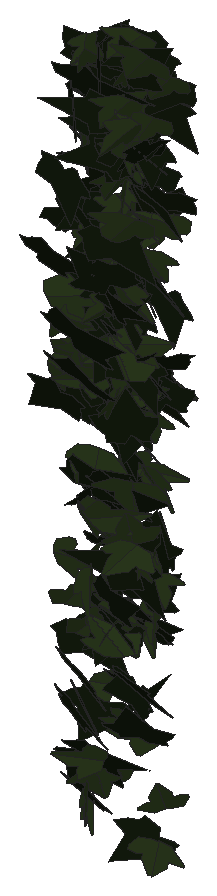
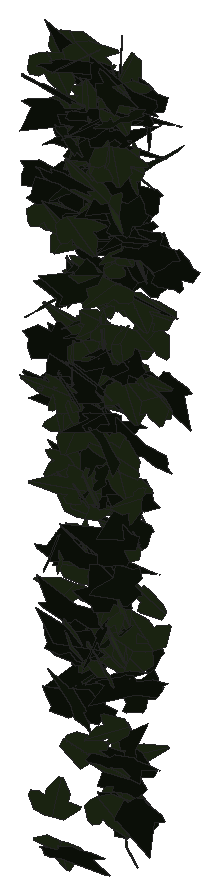
# SketchUp Ruby script. Lengths in millimetres.
U = 1.mm
M = Sketchup.active_model
def pt(a) = Geom::Point3d.new(a.map { |v| v * U })
def face(e, loops, mat)
  f = e.add_face(loops[0].map { |a| pt(a) })
  loops[1..].each { |l| e.add_face(l.map { |a| pt(a) }).erase! }
  f.material = f.back_material = mat if mat
  f
end
# faces: each face lists its corners as indices into pts; further lists are holes
def faces(e, pts, list, mat = nil) = list.each { |f| face(e, (f[0].is_a?(Array) ? f : [f]).map { |l| l.map { |i| pts[i] } }, mat) }
# xy, xz, yz: faces in a plane at the given z, y or x. An outline is a flat list of corners, or four numbers for a rectangle; further outlines are holes
def ring(l) = l.size == 4 ? [[l[0], l[1]], [l[2], l[1]], [l[2], l[3]], [l[0], l[3]]] : l.each_slice(2).to_a
def flat(e, list, mat, &to3) = list.each { |f| face(e, (f[0].is_a?(Array) ? f : [f]).map { |l| ring(l).map { |u, v| to3.(u, v) } }, mat) }
def xy(e, z, list, mat = nil) = flat(e, list, mat) { |x, y| [x, y, z] }
def xz(e, y, list, mat = nil) = flat(e, list, mat) { |x, z| [x, y, z] }
def yz(e, x, list, mat = nil) = flat(e, list, mat) { |y, z| [x, y, z] }
def lines(e, pts, list) = list.each { |a, b| e.add_line(pt(pts[a]), pt(pts[b])) }
# prism: a flat outline (further loops are holes) pulled along v
def prism(e, loops, v, mat = nil)
  f = face(e, loops, mat); d = Geom::Vector3d.new(v.map { |x| x * U })
  f.pushpull(f.normal.samedirection?(d) ? d.length : -d.length)
end
def box(e, o, s, mat = nil) = prism(e, [[o, [o[0] + s[0], o[1], o[2]], [o[0] + s[0], o[1] + s[1], o[2]], [o[0], o[1] + s[1], o[2]]]], [0, 0, s[2]], mat)
def at(x, y, z, deg = 0) = Geom::Transformation.translation(pt([x, y, z])) * Geom::Transformation.rotation(ORIGIN, Z_AXIS, deg.degrees)
def axes(o, x, y, z) = Geom::Transformation.new([*x, 0, *y, 0, *z, 0, *pt(o).to_a, 1])
def part(name) = M.definitions.add(name)
# library, detail: a bought-in or finely detailed component or shape, given as its bounding box
def library(name, o, s) = part(name).tap { |d| box(d.entities, o, s) }
def detail(e, o, s) = box(e.add_group.entities, o, s)
def put(e, d, t, mat = nil) = e.add_instance(d, t).tap { |i| i.material = mat if mat }
def group(e, t, mat = nil) = e.add_group.tap { |g| g.transformation = t; g.material = mat if mat }.entities
root = M.entities
M.materials.add("efeu1").color = [18, 25, 13]
M.materials.add("efeu2").color = [43, 57, 29]
c1 = part("ivyleaf_9")
p = [[39.1,54.8,31.7],[34.5,51.8,30.2],[-5.3,25.2,17.3],[-17.9,28.3,20.9],[-21.6,21.7,17],[-20.2,4.3,5.3],
  [-22.9,-0.3,2.5],[-17.1,-4,-0.6],[-2,-2.1,-1.2],[-0.7,-15.4,-10.1],[16.6,-22.3,-16.7],[21.1,-15.1,-12.5],
  [32.7,-10.7,-11],[46.1,-1.8,-6.6],[30.8,11.2,3.8]]
faces(c1.entities,p,[[0,1,2,3,4,5,6,7,8,9,10,11,12,13,14]],"efeu1")
c2 = part("ivyleaf_10")
p = [[0,12.8,-0.8],[-1.5,51.3,-10.9],[-4.9,51,-11.6],[-13.6,26.5,-7.3],[-13.2,15.9,-4.6],[-21.1,19.3,-7.2],
  [-29.5,16.3,-8.3],[-29.2,8.3,-6.2],[-19.7,-9.8,0.5],[-7.6,-13,4],[1,-12.2,5.8],[-0.4,51.1,-11.1],
  [-1.5,51.1,-10.9],[1,-12.4,5.9],[16.9,-12.4,3.5],[35.1,9.1,-5.1],[35,12.9,-6.1],[20.5,16.4,-4.9],
  [15.8,15,-3.8],[15.3,27.6,-7.1],[12.8,31.3,-7.8]]
faces(c2.entities,p,[[0,1,2,3,4,5,6,7,8,9,10],[11,12,0,13,14,15,16,17,18,19,20]],"efeu2")
put(root,c1,axes([2636.7,760.3,1184.7],[1.6124,-0.56615,0.10588],[-0.16714,0.05915,1.01896],[-1.08336,-0.85174,0.00038]))
put(root,c1,axes([2611.5,780.2,1231.1],[-0.08714,-0.29377,1.10403],[1.30837,-0.88957,-0.20819],[1.73659,0.65547,0.21226]))
put(root,c2,axes([2633.5,781.2,864.3],[0.85683,-0.49021,0.75163],[0.95653,-0.55892,-0.66555],[1.41486,0.67472,-0.00523]))
put(root,c1,axes([2588.5,792.1,648.9],[1.43319,-0.52934,-0.36142],[-0.54841,0.2185,-0.92039],[1.08964,0.8062,0.01214]))
put(root,c2,axes([2649.6,821.7,1130.2],[0.1327,-0.81984,-0.18916],[-0.03294,0.18837,-0.8228],[1.60097,0.07183,-0.00125]))
put(root,c1,axes([2544.3,843.4,1440.8],[-0.05269,-0.95204,0.27297],[-0.03417,-0.27255,-0.95239],[1.88462,-0.03156,-0.00964]))
put(root,c1,axes([2544.1,833.4,1099.3],[0.62412,0.12421,-0.75032],[-1.35263,-0.24082,-0.35049],[-0.51525,0.78264,0.01124]))
put(root,c2,axes([2661,844.7,884.5],[1.00057,0.45595,-0.51321],[-0.72793,-0.34225,-0.69588],[-1.08498,0.65011,-0.00641]))
put(root,c2,axes([2648.4,855.7,1540],[-0.23392,-0.64575,0.69785],[-0.07905,-0.69934,-0.65444],[1.80781,-0.11414,0.06168]))
put(root,c2,axes([2657.9,846.9,1398.1],[-1.29079,-0.56031,0.38123],[-0.57404,-0.23343,-0.87966],[1.15502,-0.74218,-0.01114]))
put(root,c1,axes([2613.9,854.3,1285.2],[0.65721,0.16862,0.86839],[-1.60064,-0.22643,0.3784],[0.52195,-0.90669,0.06699]))
put(root,c1,axes([2665.8,837.4,1077.4],[-1.67349,0.36104,-0.12202],[-0.22886,0.02832,0.95034],[0.68826,0.88728,0.01932]))
put(root,c1,axes([2620.6,846.9,1370.6],[0.06708,-0.68505,-0.71505],[0.24385,0.71265,-0.67643],[1.8688,-0.0684,0.11393]))
put(root,c1,axes([2492.5,858.1,1287.3],[0.42343,-0.24255,0.75106],[1.05325,-0.50842,-0.32813],[1.07097,0.5959,0.02575]))
put(root,c2,axes([2622.8,869.5,1114.2],[0.05493,-0.1984,0.87429],[0.54078,-0.82763,-0.19719],[1.6183,0.2833,0.03622]))
put(root,c2,axes([2580,865.8,518.5],[-0.23204,-0.13674,-0.84716],[-1.16666,-0.5849,0.18263],[-1.14288,0.62484,-0.01444]))
put(root,c2,axes([2563,867,463.3],[0.47772,-0.50253,0.66321],[0.81387,-0.51635,-0.55309],[1.35852,0.48605,0.09813]))
put(root,c1,axes([2587.5,870.7,1246.5],[0.35757,-0.24664,0.81519],[0.86605,-0.67658,-0.30958],[1.37018,0.49202,-0.01706]))
put(root,c2,axes([2573.1,872.8,1113.6],[0.33756,0.20389,-0.77068],[-1.33007,-0.3401,-0.25081],[-0.72999,0.71396,0.10061]))
put(root,c2,axes([2640.6,875.7,884.5],[-0.95042,-0.75998,-0.32042],[-0.33718,-0.26699,0.90937],[-1.53305,0.52987,-0.00136]))
put(root,c2,axes([2600,857.9,908.2],[-0.4951,-0.32007,0.79563],[0.97281,0.60975,0.41242],[-1.3106,0.57351,0.00556]))
put(root,c2,axes([2636.8,865.7,1150.4],[1.45285,0.14221,0.28272],[-0.54953,0.01077,0.77421],[0.24656,-0.81397,0.05964]))
put(root,c1,axes([2595.3,880.6,765.3],[-0.07981,-0.01194,0.86813],[0.66293,-0.79636,0.00587],[1.51356,0.34817,0.0432]))
put(root,c2,axes([2594.9,884.7,1234],[-0.18894,-0.47209,0.65973],[-0.19717,-0.65183,-0.48203],[1.53131,-0.14218,0.01934]))
put(root,c1,axes([2611.1,884.4,1469.2],[-1.27105,-0.07874,0.49317],[-0.88576,-0.20058,-0.66228],[0.34477,-0.80561,0.11669]))
put(root,c1,axes([2665.5,864.2,1102.1],[-0.0001,0.82108,0.13207],[0.00018,0.13207,-0.82108],[-1.58276,-0.00004,-0.0001]))
put(root,c2,axes([2498.8,885.8,1100.2],[-0.08474,-0.04414,-0.80849],[1.05544,-0.59165,0.00176],[-1.12284,-0.5528,0.06267]))
put(root,c1,axes([2524.4,889.7,635.8],[0.49437,-0.66612,0.54837],[0.3917,-0.50832,-0.71495],[1.59468,0.33136,0.00561]))
put(root,c2,axes([2609.1,878,701.1],[1.07533,0.55125,0.36674],[-0.5215,-0.24422,0.78923],[1.14713,-0.62777,0.01501]))
put(root,c1,axes([2518.9,889.7,1539],[-0.20167,0.03786,-0.92487],[1.53236,-0.4555,-0.11089],[-0.86914,-0.81187,0.01908]))
put(root,c1,axes([2600.6,892.9,1242.9],[-0.12424,-0.10747,0.81775],[-0.65781,-0.74124,-0.12501],[1.42525,-0.35148,0.01359]))
put(root,c1,axes([2641.9,883.7,572],[1.28895,-0.00393,0.47864],[-0.9109,0.0059,0.67726],[-0.01259,-0.8293,0.00255]))
put(root,c1,axes([2627.8,895.5,631.9],[0.61513,-0.71398,-0.4213],[0.31013,-0.38865,0.78366],[-1.54699,-0.36181,-0.01042]))
put(root,c1,axes([2636.2,883.3,1158.1],[-0.16363,-0.83193,-0.3462],[0.0873,0.34328,-0.83631],[1.71274,-0.09698,0.00956]))
put(root,c1,axes([2614.1,898.9,1050.6],[-0.30402,-0.84049,0.4832],[-0.08675,-0.48266,-0.85462],[1.84308,-0.16136,0.03948]))
put(root,c2,axes([2614.8,888.1,1551.9],[-0.81112,-0.66346,0.40932],[-0.30664,-0.38146,-0.78606],[1.45163,-0.45129,0.06267]))
put(root,c2,axes([2637.9,879.6,962.2],[-1.64954,-0.50452,-0.01723],[0.03126,0.00604,-1.00286],[0.96025,-0.86687,0.00304]))
put(root,c2,axes([2615.9,886.7,1261.3],[-0.83842,0.17875,-0.66675],[1.00765,-0.42003,-0.46243],[-0.84299,-0.67985,0.11039]))
put(root,c2,axes([2515,872.2,1224.9],[0.4771,0.06473,-0.91337],[1.62568,0.3246,0.25744],[0.62777,-0.88978,0.02747]))
put(root,c1,axes([2591.7,887.1,1526],[-0.97841,0.14637,0.63984],[-1.24803,-0.07931,-0.50873],[-0.05415,-0.81694,0.16403]))
put(root,c2,axes([2538.2,894.7,1469.3],[-0.2072,0.51045,-0.77588],[0.32854,-0.75646,-0.52189],[-1.73677,-0.20399,-0.00616]))
put(root,c1,axes([2552.9,894.8,877.4],[0.44546,-0.56495,0.55341],[0.4044,-0.51099,-0.61151],[1.44979,0.31612,0.00053]))
put(root,c1,axes([2594.9,890,928.6],[-0.04633,-0.21976,0.96131],[1.4186,-0.63368,-0.12599],[1.22875,0.7233,0.1817]))
put(root,c1,axes([2626.7,889.4,824.4],[-0.70576,-0.27346,-0.68713],[-0.93529,-0.4833,0.45756],[-1.0518,0.61326,0.05419]))
put(root,c1,axes([2552.1,903.2,1331.5],[-0.10862,-0.68672,0.7197],[-0.08723,-0.7183,-0.68902],[1.89122,-0.07257,0.00955]))
put(root,c2,axes([2625.2,896.7,843.3],[-0.09769,-0.08634,0.89803],[1.38659,-0.53447,-0.00975],[1.01267,0.72349,0.09998]))
put(root,c1,axes([2564.7,895.9,1578.6],[-0.07357,0.26157,0.84229],[-0.3734,-0.82453,0.24705],[1.63651,-0.17637,0.09423]))
put(root,c2,axes([2624.9,886.8,1491.4],[-1.03187,-0.61606,0.11639],[-0.12879,-0.09547,-0.82057],[1.18625,-0.54625,0.01215]))
put(root,c2,axes([2589.7,896.7,1161],[0.27726,0.38897,-0.73894],[-0.80704,-0.61174,-0.40561],[-1.36914,0.43935,0.08945]))
put(root,c2,axes([2617.3,892.6,1418.6],[-0.00447,0.68767,-0.46304],[-0.19118,-0.45986,-0.68245],[-1.56618,0.05417,0.08463]))
put(root,c1,axes([2556,889.8,931.8],[-0.4108,-0.03871,0.90493],[1.41963,-0.53531,0.15502],[0.97787,0.76087,0.1551]))
put(root,c1,axes([2655.2,891.2,1500.4],[-0.24583,0.55464,-0.60963],[0.25304,-0.59497,-0.56947],[-1.54804,-0.18533,0.00373]))
put(root,c2,axes([2521.8,873.6,1194.5],[-0.39813,-0.57342,-0.79102],[0.68733,0.70627,-0.60749],[1.72773,-0.41311,0.05939]))
put(root,c1,axes([2541.4,887.3,508.7],[1.29997,0.23669,-0.56849],[1.01756,0.19327,0.72287],[0.58146,-0.86739,0.00594]))
put(root,c2,axes([2572.1,901.8,1296.4],[-0.15489,0.21723,0.77842],[0.10988,-0.77879,0.22337],[1.53416,0.07771,0.06259]))
put(root,c1,axes([2585.8,905.8,1149.5],[-0.61849,-0.71147,0.46147],[-0.27678,-0.44012,-0.78096],[1.59006,-0.35336,0.04356]))
put(root,c1,axes([2617.7,884,1466.3],[-1.25077,0.53031,0.365],[-0.57221,0.2084,-0.84411],[-1.08342,-0.72229,0.02444]))
put(root,c2,axes([2536.3,894.4,1321.4],[0.72371,-0.70038,0.1872],[0.16782,-0.16514,-0.79695],[1.36952,0.39035,-0.00127]))
put(root,c1,axes([2626.5,884.6,1394.6],[1.30464,-0.264,-0.36948],[-0.64215,0.15167,-0.73435],[0.57843,0.76382,0.01811]))
put(root,c1,axes([2615.4,895.4,828.7],[-0.60342,-0.13686,-0.90242],[1.664,0.22871,-0.34187],[0.49868,-0.92875,0.04879]))
put(root,c2,axes([2598.5,894.4,1429.9],[-0.45056,-0.80112,0.11737],[-0.08862,-0.10861,-0.83525],[1.53842,-0.24088,-0.01374]))
put(root,c1,axes([2598.4,903.8,1323],[-1.25383,-0.31045,0.38865],[-0.63392,-0.20371,-0.72733],[0.70311,-0.73727,0.03731]))
put(root,c1,axes([2622.9,907.3,1137],[0.36946,-0.49314,0.77936],[0.52436,-0.72906,-0.52994],[1.67511,0.33698,-0.00601]))
put(root,c2,axes([2539.8,904.1,879.7],[-0.21889,0.15651,-0.96489],[1.18442,-0.73749,-0.1938],[-1.43464,-0.63274,-0.01278]))
put(root,c1,axes([2524.3,893.4,1554.2],[0.80138,-0.18618,0.85758],[1.50624,-0.33041,-0.46032],[0.72161,0.89643,0.00844]))
put(root,c1,axes([2604.9,890.1,646.9],[1.49151,-0.23894,0.08391],[0.1569,-0.01732,-0.81927],[0.45572,0.78798,0.00744]))
put(root,c1,axes([2532.5,903.4,434.9],[1.2243,-0.43889,-0.06623],[0.11576,-0.02835,0.77867],[-0.83678,-0.64607,0.01082]))
put(root,c1,axes([2610.8,884.6,1466.2],[-0.77933,-0.26051,0.67771],[1.04371,0.39895,0.4847],[-0.90561,0.68397,-0.02459]))
put(root,c1,axes([2601.8,907.8,1034.8],[0.38992,-0.61087,0.62806],[0.52511,-0.5672,-0.64168],[1.58262,0.3387,0.05817]))
put(root,c2,axes([2623.5,894.7,1175.1],[0.77944,-0.11452,-0.71294],[1.34701,-0.09875,0.42243],[-0.27231,-0.81624,0.04892]))
put(root,c2,axes([2649.2,892.5,1325],[-1.43005,-0.2407,-0.27073],[0.49402,0.07712,-0.78898],[0.48092,-0.79494,0.00544]))
put(root,c1,axes([2576.8,892.4,1253.1],[-0.73984,0.35747,0.62926],[-1.10494,0.27243,-0.51342],[-0.82235,-0.68766,0.12371]))
put(root,c2,axes([2496.1,904.7,796.6],[0.42331,-0.21006,-0.8027],[1.20912,-0.49143,0.30464],[-1.01575,-0.67253,0.02811]))
put(root,c1,axes([2578.1,911.4,1486.1],[-0.28995,-0.06419,0.88028],[-1.35087,-0.52204,-0.16091],[0.99843,-0.72496,0.03793]))
put(root,c2,axes([2585.2,893.2,701.3],[0.14791,-0.8532,0.33575],[-0.08992,0.33278,0.85659],[-1.74271,-0.08959,-0.0157]))
put(root,c1,axes([2551.9,897,551.9],[0.20098,-0.58066,0.51564],[-0.01396,0.51962,0.58664],[-1.47788,-0.08387,0.06458]))
put(root,c1,axes([2623.8,883.8,1242.9],[-1.05324,0.68611,-0.1935],[-0.23137,0.15055,0.88148],[1.33687,0.5666,0.00011]))
put(root,c2,axes([2560.3,895.6,475.5],[-1.0088,-0.61644,-0.22224],[0.28649,0.16365,-0.81296],[1.21376,-0.55097,0.00718]))
put(root,c2,axes([2554.9,901,973.7],[1.5478,0.10424,-0.01068],[-0.02017,-0.0013,-0.81991],[-0.1984,0.81333,0.00006]))
put(root,c2,axes([2543,899.8,1254.8],[-1.3826,-0.1609,0.31255],[-0.55635,-0.12205,-0.74228],[0.37161,-0.78137,0.05159]))
put(root,c2,axes([2647.4,903.4,1373],[0.98495,0.59596,-0.26554],[-0.32446,-0.20364,-0.78929],[-1.19859,0.54486,-0.00455]))
put(root,c2,axes([2596.1,911.6,1378.7],[-0.60535,-0.61315,0.55252],[-0.09267,-0.57716,-0.66852],[1.56811,-0.27081,0.17379]))
put(root,c2,axes([2651,898.4,1373.9],[-1.65444,-0.17236,0.04788],[-0.08929,-0.00958,-0.88622],[0.32853,-0.87056,0.00027]))
put(root,c2,axes([2548.3,888.7,1615.3],[0.0006,-0.58195,-0.70668],[0.39682,0.68816,-0.5666],[1.69651,-0.16075,0.13278]))
put(root,c1,axes([2562.9,916.1,732.1],[0.27707,-0.77645,0.53545],[0.3976,-0.50179,-0.78444],[1.75047,0.23688,0.09342]))
put(root,c2,axes([2514.6,899.9,733.6],[-0.86301,-0.75182,0.26332],[0.25519,0.22664,0.87798],[-1.49446,0.47286,-0.00214]))
put(root,c2,axes([2641.5,901.4,1624.6],[-1.47567,-0.11096,0.38201],[-0.70729,-0.09648,-0.78232],[0.27008,-0.85896,0.03852]))
put(root,c1,axes([2597.9,910.3,720.3],[-1.45525,-0.2128,0.03225],[-0.05372,-0.01885,-0.79362],[0.40608,-0.76508,0.01058]))
put(root,c2,axes([2630.4,885,1474.4],[-0.31683,0.55936,0.8349],[-0.41595,0.80588,-0.58349],[-1.86687,-0.27448,-0.01169]))
put(root,c1,axes([2590.8,915.7,1477.9],[0.32841,-0.63262,0.66271],[0.87842,-0.52251,-0.61897],[1.50625,0.44265,0.21648]))
put(root,c2,axes([2531.6,916.8,413.9],[0.57883,-0.34575,0.73459],[0.92056,-0.55287,-0.46047],[1.24103,0.57136,-0.00105]))
put(root,c2,axes([2548.7,910.9,1333.4],[0.57967,0.63822,-0.40303],[-0.27642,-0.37693,-0.70665],[-1.40974,0.33634,-0.02716]))
put(root,c2,axes([2534,920.1,697.3],[0.17432,-0.07272,0.94033],[1.27644,-0.65921,-0.11631],[1.26201,0.6768,-0.01225]))
put(root,c2,axes([2644.6,908.2,1526.8],[-1.21799,-0.4633,0.24883],[-0.33905,-0.17777,-0.78917],[0.9417,-0.66323,0.0377]))
put(root,c1,axes([2502.9,891.9,1349.3],[0.26248,0.13266,-0.84326],[0.32224,0.83297,0.15873],[1.59235,-0.19043,0.10688]))
put(root,c2,axes([2608.5,895,1463.5],[0.6674,0.4968,0.56306],[0.37714,0.53818,-0.59826],[-1.37845,0.38778,0.10893]))
put(root,c1,axes([2628.9,909.2,1088.7],[0.51454,-0.6387,0.36456],[-0.11388,0.36803,0.68914],[-1.39502,-0.26562,0.07821]))
put(root,c2,axes([2534.2,902.2,693],[-0.60831,-0.74599,0.40367],[0.30536,0.37041,0.81158],[-1.58515,0.35763,0.00143]))
put(root,c1,axes([2630.9,915.7,1411.9],[0.68928,-0.79476,0.17443],[0.17885,-0.14879,-0.87308],[1.53822,0.37343,0.02335]))
put(root,c1,axes([2633.2,917.4,1485.6],[-0.34887,-0.80207,-0.03123],[0.01682,0.03001,-0.82274],[1.52756,-0.18351,0.00193]))
put(root,c1,axes([2602.4,922,1213],[-0.21845,-0.79669,0.27399],[0.0454,-0.27949,-0.80267],[1.60278,-0.10067,0.06008]))
put(root,c1,axes([2554.9,920.5,1352.3],[-1.26487,-0.3726,0.30722],[-0.43938,-0.21391,-0.75885],[0.80728,-0.70023,0.06834]))
put(root,c2,axes([2608.2,911.2,1158.8],[-1.04878,-0.46259,0.30455],[-0.4475,-0.19358,-0.71948],[0.95438,-0.59912,-0.00268]))
put(root,c1,axes([2624.1,923.5,1243.9],[0.00859,-0.20055,0.79906],[0.01179,-0.79904,-0.20058],[1.5679,0.00711,-0.00287]))
put(root,c2,axes([2598.6,903,709.8],[-1.05776,-0.73185,-0.37562],[0.43859,0.29664,-0.91896],[1.50292,-0.60165,0.00382]))
put(root,c1,axes([2668.5,910.2,1161.8],[-0.03704,0.71355,-0.61813],[-0.1191,-0.61788,-0.71129],[-1.79278,0.0263,0.06002]))
put(root,c2,axes([2626.2,921.8,820.6],[-0.03258,-0.07094,0.79621],[-0.65766,-0.71749,-0.07135],[1.37187,-0.34564,-0.0153]))
put(root,c2,axes([2572.1,899.2,741.3],[-0.75518,-0.49368,-0.65916],[0.84721,0.48701,-0.63271],[1.31865,-0.59562,0.02901]))
put(root,c2,axes([2611.5,895.1,1547.8],[0.26382,0.49802,0.65345],[-0.00989,0.6632,-0.50435],[-1.56362,0.07983,0.11344]))
put(root,c1,axes([2537.3,889.7,909.4],[0.65747,0.49988,0.72766],[0.69587,0.63021,-0.60652],[-1.52931,0.50166,0.03685]))
put(root,c1,axes([2523.9,899.5,1376.2],[0.41068,-0.20512,-0.76242],[-0.37167,0.75196,-0.25757],[1.45595,0.24982,0.1493]))
put(root,c2,axes([2642.7,914.8,966.8],[-0.94871,0.52672,-0.46065],[0.58254,-0.34447,-0.7251],[-1.19757,-0.58483,0.01221]))
put(root,c1,axes([2666,911.1,1418.1],[0.61654,0.5127,-0.62044],[-0.63476,-0.52318,-0.60647],[-1.39412,0.46495,0.00174]))
put(root,c1,axes([2580.6,928,996.3],[0.17248,-0.70819,0.53318],[0.13668,-0.52833,-0.71396],[1.68158,0.11558,0.00334]))
put(root,c2,axes([2543.8,898.6,1461.8],[-0.31791,0.36092,-0.85968],[-0.66984,0.78434,0.39768],[1.6432,0.38956,-0.00421]))
put(root,c2,axes([2521.5,920.4,1163.4],[1.01892,-0.46618,0.2947],[0.40983,-0.20142,-0.70983],[0.96634,0.57697,-0.00969]))
put(root,c1,axes([2596.6,914.8,1587.9],[-0.65354,0.36354,0.87223],[1.14045,-0.63381,0.50008],[1.39061,0.69064,-0.0002]))
put(root,c2,axes([2529.4,896.4,945.4],[0.17771,0.07205,-0.92569],[0.57571,0.87724,0.09879],[1.67069,-0.30995,0.06442]))
put(root,c2,axes([2567.9,899.7,1148.3],[0.05645,0.43063,0.7255],[-0.31003,0.71521,-0.41787],[-1.57547,-0.12531,0.10822]))
put(root,c2,axes([2502.2,914.5,1120.5],[-1.25943,0.05436,-0.61325],[1.15792,-0.08004,-0.66361],[-0.17932,-0.89865,0.02201]))
put(root,c1,axes([2578.6,912.9,1119.5],[0.02372,-0.54744,-0.54993],[-0.04696,0.54944,-0.54751],[1.47605,0.02628,-0.00858]))
put(root,c1,axes([2585,933.7,961.5],[-0.12081,-0.47882,0.77083],[0.14462,-0.7728,-0.47379],[1.72097,0.03133,0.09392]))
put(root,c1,axes([2528.4,901.8,1437],[1.46476,0.48589,0.25316],[0.38092,0.15701,-0.90984],[-0.97067,0.79484,0.02497]))
put(root,c1,axes([2645.1,918.2,1491.6],[-1.08937,0.52634,-0.30745],[0.38768,-0.23235,-0.77699],[-1.09342,-0.60677,0.03083]))
put(root,c2,axes([2565.6,917.9,737.7],[-1.34851,-0.45588,0.23631],[-0.36775,-0.13639,-0.84248],[0.90544,-0.73436,0.00977]))
put(root,c1,axes([2575.6,917.4,1373.3],[-0.58515,-0.55281,-0.6408],[0.60183,0.55735,-0.63254],[1.49401,-0.44103,0.00383]))
put(root,c2,axes([2638.8,931.1,833.7],[-0.00482,0.18198,-0.75905],[-0.14087,-0.75569,-0.18093],[-1.47887,0.07139,0.01971]))
put(root,c1,axes([2657.4,927.2,1381],[0.40097,0.17972,0.82727],[-1.38191,-0.39996,0.27181],[0.82841,-0.75419,0.05299]))
put(root,c1,axes([2618.3,912.2,594.5],[-0.1952,0.82329,0.28892],[-0.03529,-0.2929,0.82805],[1.66019,0.09057,0.05157]))
put(root,c2,axes([2629.9,906.7,1145.9],[-0.03763,-0.65704,-0.66897],[-0.02333,0.66924,-0.65694],[1.78441,-0.0051,-0.0227]))
put(root,c1,axes([2523.7,930.4,1161.9],[0.07867,-0.22693,0.8247],[0.63859,-0.75519,-0.22461],[1.49743,0.33397,0.05246]))
put(root,c2,axes([2531.9,920.7,1125.5],[-1.11338,-0.63572,0.1325],[-0.15679,-0.10424,-0.86387],[1.22591,-0.59069,0.00985]))
put(root,c1,axes([2513.5,913.8,1031],[-1.07821,0.52634,0.60272],[0.84433,-0.408,0.77329],[1.26744,0.71955,-0.0024]))
put(root,c2,axes([2643.6,921,378.5],[1.48061,0.01551,0.01079],[0.02044,0.00255,-0.77811],[-0.02959,0.77803,0.00233]))
put(root,c1,axes([2536.1,925.1,1197.9],[0.32899,-0.81229,-0.14974],[-0.04375,0.14819,-0.83044],[1.57138,0.17419,0.00823]))
put(root,c2,axes([2602.6,927.6,1633.6],[-1.03433,-0.41349,0.48166],[-0.47883,-0.44184,-0.66318],[1.10921,-0.57631,0.16286]))
put(root,c1,axes([2533,916,479.2],[0.90332,0.30534,-0.65791],[-1.10003,-0.31578,-0.56353],[-0.83395,0.74726,0.03069]))
put(root,c2,axes([2663,921.4,1592.8],[-1.28745,-0.40888,0.27236],[-0.47143,-0.11641,-0.78997],[0.80747,-0.71989,-0.02695]))
put(root,c1,axes([2544.7,929.4,1192.8],[-0.24487,-0.90428,-0.14311],[0.06148,0.13995,-0.91331],[1.74136,-0.1321,0.01212]))
put(root,c2,axes([2591.3,932.4,1120.8],[0.85363,-0.38571,0.7117],[1.09241,-0.4222,-0.59054],[1.08637,0.72762,0.0346]))
put(root,c1,axes([2552.3,916.9,1346],[0.04797,0.01828,0.98426],[1.84957,-0.15753,-0.02196],[0.29888,0.9719,-0.02207]))
put(root,c2,axes([2554,924,1027],[-0.88394,0.00375,0.71478],[1.36011,0.01936,0.46426],[-0.027,0.8522,-0.01369]))
put(root,c2,axes([2564.2,929.5,472.9],[-0.84822,-0.63806,0.41851],[-0.39926,-0.36353,-0.77765],[1.39631,-0.49155,0.03187]))
put(root,c2,axes([2631.3,908.5,1090.8],[-0.01697,-0.05803,0.78167],[0.39511,0.75363,0.05832],[-1.4385,0.20768,0.0068]))
put(root,c1,axes([2543.2,906.7,1405.4],[0.12494,0.26502,-0.77192],[-0.13548,0.77332,0.25945],[1.54738,0.04631,0.08504]))
put(root,c2,axes([2607.3,932.1,1085],[-0.24701,-0.76739,0.29801],[-0.10644,-0.29277,-0.77827],[1.56314,-0.1412,-0.00591]))
put(root,c2,axes([2600.5,935.8,937.1],[0.19318,-0.19936,-0.74319],[0.90427,-0.57341,0.21871],[-1.15191,-0.48357,0.04705]))
put(root,c1,axes([2532.8,932.7,883.5],[0.91469,-0.42717,0.63079],[0.8851,-0.42622,-0.64297],[1.14838,0.66874,-0.00687]))
put(root,c2,axes([2531.3,931.8,1598.8],[0.98484,0.47535,-0.46251],[-0.69468,-0.28569,-0.70199],[-1.0539,0.63251,0.03052]))
put(root,c1,axes([2514.7,923.3,679.3],[-0.01751,-0.64966,-0.7024],[0.33013,0.68965,-0.64015],[1.79076,-0.13349,0.11114]))
put(root,c1,axes([2568,914.9,745.2],[0.48094,-0.34185,-0.84202],[-0.95453,0.67635,-0.42511],[1.44231,0.5616,-0.00057]))
put(root,c2,axes([2622.3,937,741],[0.99017,-0.48796,0.49163],[0.66622,-0.34535,-0.71322],[1.13757,0.62699,-0.01023]))
put(root,c2,axes([2648.8,936.1,442.1],[-0.84737,-0.63436,-0.32306],[-0.34452,-0.26763,0.775],[-1.31033,0.4806,0.00515]))
put(root,c1,axes([2537.7,922.3,1577.6],[-1.2759,0.37527,0.63127],[1.04918,-0.30757,0.76828],[0.92344,0.86795,-0.00068]))
put(root,c2,axes([2558.6,924.2,1278.9],[1.28648,0.47955,0.41645],[0.61204,0.26604,-0.82832],[-1.04239,0.74805,0.02762]))
put(root,c1,axes([2631.2,938.6,383],[-1.42327,-0.29792,0.1534],[-0.2714,-0.05653,-0.80499],[0.57713,-0.76131,-0.00026]))
put(root,c1,axes([2603.8,939.8,1520.4],[-0.44794,-0.07648,0.83036],[-1.50429,-0.2545,-0.24748],[0.50577,-0.8247,-0.00064]))
put(root,c2,axes([2658.2,934.6,1366.9],[-1.14145,-0.42821,0.35565],[-0.37244,-0.32723,-0.724],[0.99178,-0.61572,0.13744]))
put(root,c2,axes([2633.4,926.7,1080.2],[-0.56798,-0.73939,-0.21711],[0.17904,0.19612,-0.79723],[1.45565,-0.31263,0.01334]))
put(root,c1,axes([2544.8,942.2,685.5],[-0.67424,-0.71717,0.1147],[-0.08319,-0.10633,-0.79986],[1.37977,-0.35686,0.00782]))
put(root,c2,axes([2610.6,927.9,548.3],[0.64766,-0.06903,-0.8921],[-1.62403,0.2621,-0.34578],[0.51231,0.91812,0.03164]))
put(root,c2,axes([2539.8,931.8,785.7],[-0.83217,0.57651,-0.30835],[0.36559,-0.2413,-0.72354],[-1.18937,-0.47754,-0.00665]))
put(root,c1,axes([2657,923.1,1084.3],[-1.70104,0.11847,0.07707],[0.14135,-0.0261,0.90145],[0.22885,0.89672,0.01605]))
put(root,c1,axes([2630.3,934.9,1117.9],[-1.22465,0.50451,-0.44426],[0.67638,-0.26671,-0.81762],[-1.08598,-0.73504,-0.00825]))
put(root,c2,axes([2512.9,936.7,1025],[-0.09227,0.01227,0.86142],[1.60741,-0.16948,0.04995],[0.32336,0.84597,-0.00249]))
put(root,c2,axes([2614.2,928.7,1044.8],[-1.55313,-0.18859,-0.13277],[0.24503,0.03255,-0.83757],[0.3642,-0.82615,-0.00269]))
put(root,c2,axes([2532.4,933,811.9],[0.20838,-0.77654,-0.049],[-0.01251,0.04856,-0.78422],[1.4808,0.10969,0.00027]))
put(root,c1,axes([2542,926.6,1077.8],[0.25988,-0.44334,-0.72006],[0.52186,0.71319,-0.38711],[1.52238,-0.16879,0.25562]))
put(root,c1,axes([2642.1,947.2,1235.7],[-0.06362,-0.93443,0.2435],[-0.0529,-0.24261,-0.93485],[1.83704,-0.03935,-0.01849]))
put(root,c1,axes([2604.4,941.9,1266.9],[0.82263,-0.67212,0.32669],[0.32805,-0.27755,-0.79909],[1.38392,0.46531,-0.00477]))
put(root,c1,axes([2625.2,930.1,835.5],[-1.22259,-0.06086,0.45253],[0.86807,-0.12191,0.63107],[0.04047,0.77626,0.13459]))
put(root,c1,axes([2539,943.8,560.4],[-1.33564,-0.49269,-0.06541],[0.10137,0.03797,-0.85747],[0.94047,-0.7038,-0.00047]))
put(root,c2,axes([2608.5,943.4,709.4],[0.86251,-0.30991,0.60783],[0.9301,-0.36174,-0.54881],[0.90611,0.66632,-0.01523]))
put(root,c1,axes([2586.3,944.8,1277.4],[0.80442,-0.77344,0.38973],[0.43576,-0.31845,-0.88029],[1.58968,0.47867,0.04409]))
put(root,c1,axes([2600.1,944.4,1626.3],[0.01727,-0.83001,0.03306],[0.00102,-0.03305,-0.83006],[1.58094,0.00909,0.00017]))
put(root,c2,axes([2619.3,932.2,794.3],[1.26064,0.43416,0.28408],[0.45619,0.15251,-0.79197],[-0.87576,0.7044,-0.00362]))
put(root,c2,axes([2588.6,932,1580.3],[0.00794,-0.81409,-0.25696],[0.1155,0.2566,-0.81195],[1.62062,-0.0143,0.05912]))
put(root,c1,axes([2560.4,930,1146.8],[-1.47159,-0.1518,0.34435],[0.66273,0.00976,0.78621],[-0.27158,0.84637,0.0527]))
put(root,c1,axes([2609,936.9,1137],[-1.5949,0.35325,0.03998],[-0.07064,0.01487,-0.90942],[-0.67291,-0.83883,0.00071]))
put(root,c1,axes([2590.9,936.8,1094.5],[-0.00127,0.00453,-0.90717],[1.63214,0.29587,0.00085],[0.56311,-0.85757,-0.0045]))
put(root,c1,axes([2564.9,918.7,1036.5],[0.03003,0.65304,0.55848],[-0.02856,0.5587,-0.65288],[-1.63514,0.00224,0.02166]))
put(root,c2,axes([2523.5,946.9,728.5],[0.3341,-0.41955,-0.66535],[0.58127,-0.59187,0.4538],[-1.37957,-0.35099,0.03007]))
put(root,c2,axes([2542.9,936.2,1495],[-1.09354,-0.57608,0.05605],[-0.08358,-0.03537,-0.81361],[1.09839,-0.57622,-0.0061]))
put(root,c2,axes([2538.9,940.6,1579.5],[-0.50985,-0.79434,0.18451],[-0.07502,-0.18137,-0.83805],[1.55022,-0.27003,0.02013]))
put(root,c1,axes([2629.2,949.9,1612.1],[-1.25867,-0.30761,0.44171],[-0.68281,-0.26973,-0.72501],[0.7637,-0.74815,0.07978]))
put(root,c1,axes([2611.4,944.1,705.5],[1.15615,-0.47511,0.2831],[-0.41527,0.18054,0.77117],[-0.96722,-0.64543,0.00731]))
put(root,c2,axes([2564.8,940.7,1428.6],[1.04452,-0.22672,-0.62542],[1.08345,-0.25944,0.59361],[-0.65509,-0.7906,-0.01544]))
put(root,c1,axes([2594.4,944.6,705.8],[-0.03717,-0.14758,0.80337],[1.08004,-0.58043,-0.09283],[1.11809,0.55577,0.11638]))
put(root,c1,axes([2517.7,952.1,1563.9],[-0.15342,-0.77865,0.31745],[0.28499,-0.3271,-0.7643],[1.57478,-0.01667,0.16924]))
put(root,c1,axes([2631.1,935,1535.3],[-0.40675,-0.39699,-0.75706],[0.69198,0.66404,-0.45085],[1.47242,-0.42174,0.00275]))
put(root,c1,axes([2537.5,944.6,805.8],[1.44571,-0.06089,-0.07264],[0.13813,-0.00362,0.76205],[-0.11602,-0.76307,0.00218]))
put(root,c2,axes([2521.6,954.1,1214.8],[-0.05982,-0.25352,0.78401],[0.534,-0.74099,-0.22835],[1.47448,0.25807,0.11451]))
put(root,c2,axes([2578.8,945.4,978.3],[0.5608,-0.72997,0.22228],[0.18558,-0.20031,-0.78706],[1.44036,0.31002,0.01486]))
put(root,c1,axes([2656.2,932.4,827.6],[-0.21893,-0.49954,0.70126],[0.44665,0.66251,0.51043],[-1.57659,0.25706,0.04723]))
put(root,c2,axes([2570.3,938.5,1466.1],[-1.03943,0.66778,-0.05249],[-0.07717,0.03465,0.86262],[1.27251,0.54757,0.00943]))
put(root,c1,axes([2545.8,950.3,1610.9],[-0.81735,0.26931,-0.65713],[0.56463,-0.62969,-0.45195],[-1.22802,-0.46877,0.22957]))
put(root,c1,axes([2635.5,945.8,1435.7],[-1.58823,0.00371,0.04795],[-0.09125,0.00106,-0.83451],[-0.00717,-0.83588,-0.00085]))
put(root,c1,axes([2610.4,937.7,753.2],[-0.77226,0.25126,0.66866],[1.06229,-0.36837,0.47713],[0.84836,0.68998,0.01123]))
put(root,c1,axes([2653.7,950.7,1572.4],[-1.47134,-0.18213,-0.23459],[0.51432,-0.16004,-0.76631],[0.23445,-0.79189,0.20882]))
put(root,c2,axes([2530.1,939.2,1222.5],[-1.41358,-0.32233,-0.02965],[0.05173,0.01184,-0.80967],[0.61388,-0.74324,-0.00004]))
put(root,c2,axes([2541.6,926.9,599.1],[0.15637,0.20169,0.73887],[0.29287,0.72361,-0.21463],[-1.42794,0.1705,0.03689]))
put(root,c2,axes([2615.5,944.8,1099],[-0.17333,-0.04313,-0.87343],[1.56084,-0.30906,-0.07025],[-0.57777,-0.82198,0.07224]))
put(root,c1,axes([2556.7,938.6,1549.9],[0.61847,-0.6411,-0.46545],[-0.11591,0.48138,-0.70556],[1.50334,0.30086,0.13709]))
put(root,c1,axes([2572.6,954.1,1558.2],[-1.1634,-0.542,0.13138],[-0.18797,-0.08663,-0.81696],[1.04462,-0.61921,-0.00069]))
put(root,c2,axes([2554.9,943.7,685.4],[1.25347,-0.52729,-0.20055],[0.30721,-0.11926,0.84365],[-1.02878,-0.67806,0.00757]))
put(root,c2,axes([2576.1,927.1,1223.5],[0.49579,0.49924,-0.67993],[0.41196,0.64822,0.55889],[1.55165,-0.33162,0.06887]))
put(root,c1,axes([2613,944.4,1112.5],[0.79064,-0.40758,0.66623],[-0.90454,0.46689,0.58198],[-1.17953,-0.63124,0.00028]))
put(root,c2,axes([2593.9,932.7,954.8],[0.04775,-0.0054,0.92465],[1.27515,0.63759,-0.01446],[-1.21283,0.67014,0.0212]))
put(root,c2,axes([2525.1,954.6,1424.1],[0.50508,-0.66728,0.49053],[0.34138,-0.45656,-0.71811],[1.53878,0.32031,-0.0017]))
put(root,c2,axes([2566.1,929.6,1227.4],[0.11651,-0.33489,-0.79122],[-0.26012,0.77933,-0.34043],[1.61436,0.14974,0.00225]))
put(root,c1,axes([2497.5,956.6,1413.6],[0.3435,-0.54099,0.65103],[0.54215,-0.58802,-0.5676],[1.51704,0.33264,0.05543]))
put(root,c1,axes([2503.4,944.5,842.9],[1.22066,-0.47632,0.05544],[0.09004,-0.02929,-0.79888],[0.9082,0.6431,0.00468]))
put(root,c2,axes([2602.2,949.2,1370.6],[-0.75517,-0.64724,0.32465],[-0.35168,-0.26744,-0.75901],[1.33247,-0.4374,-0.01633]))
